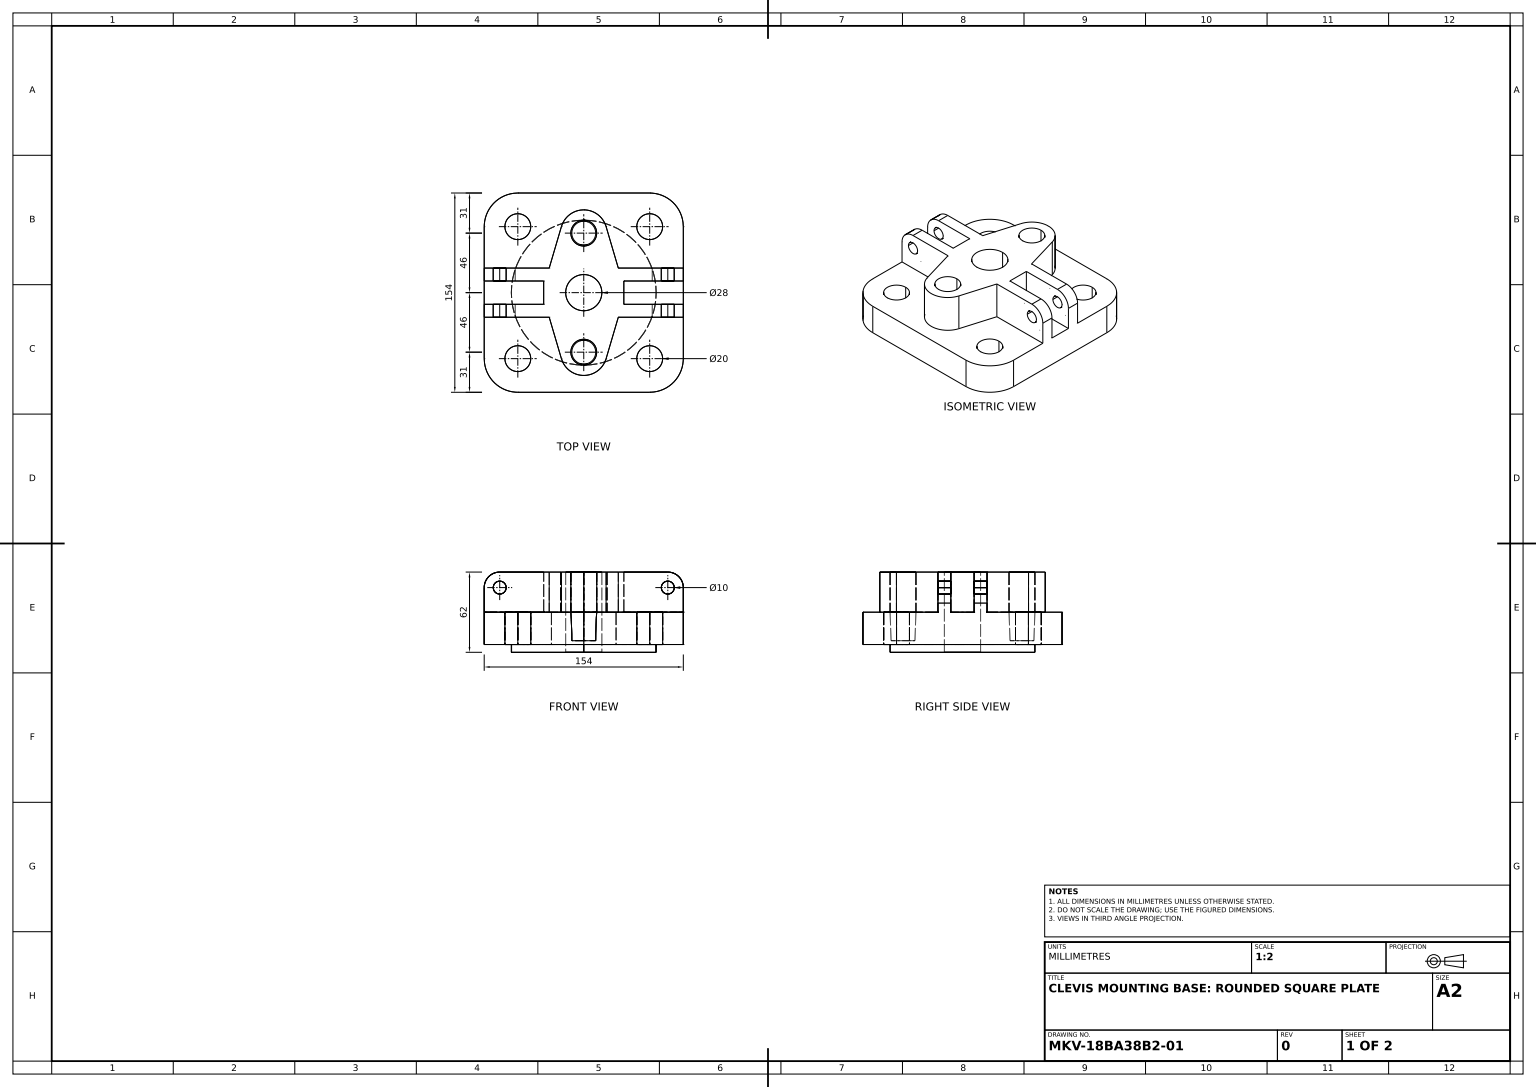
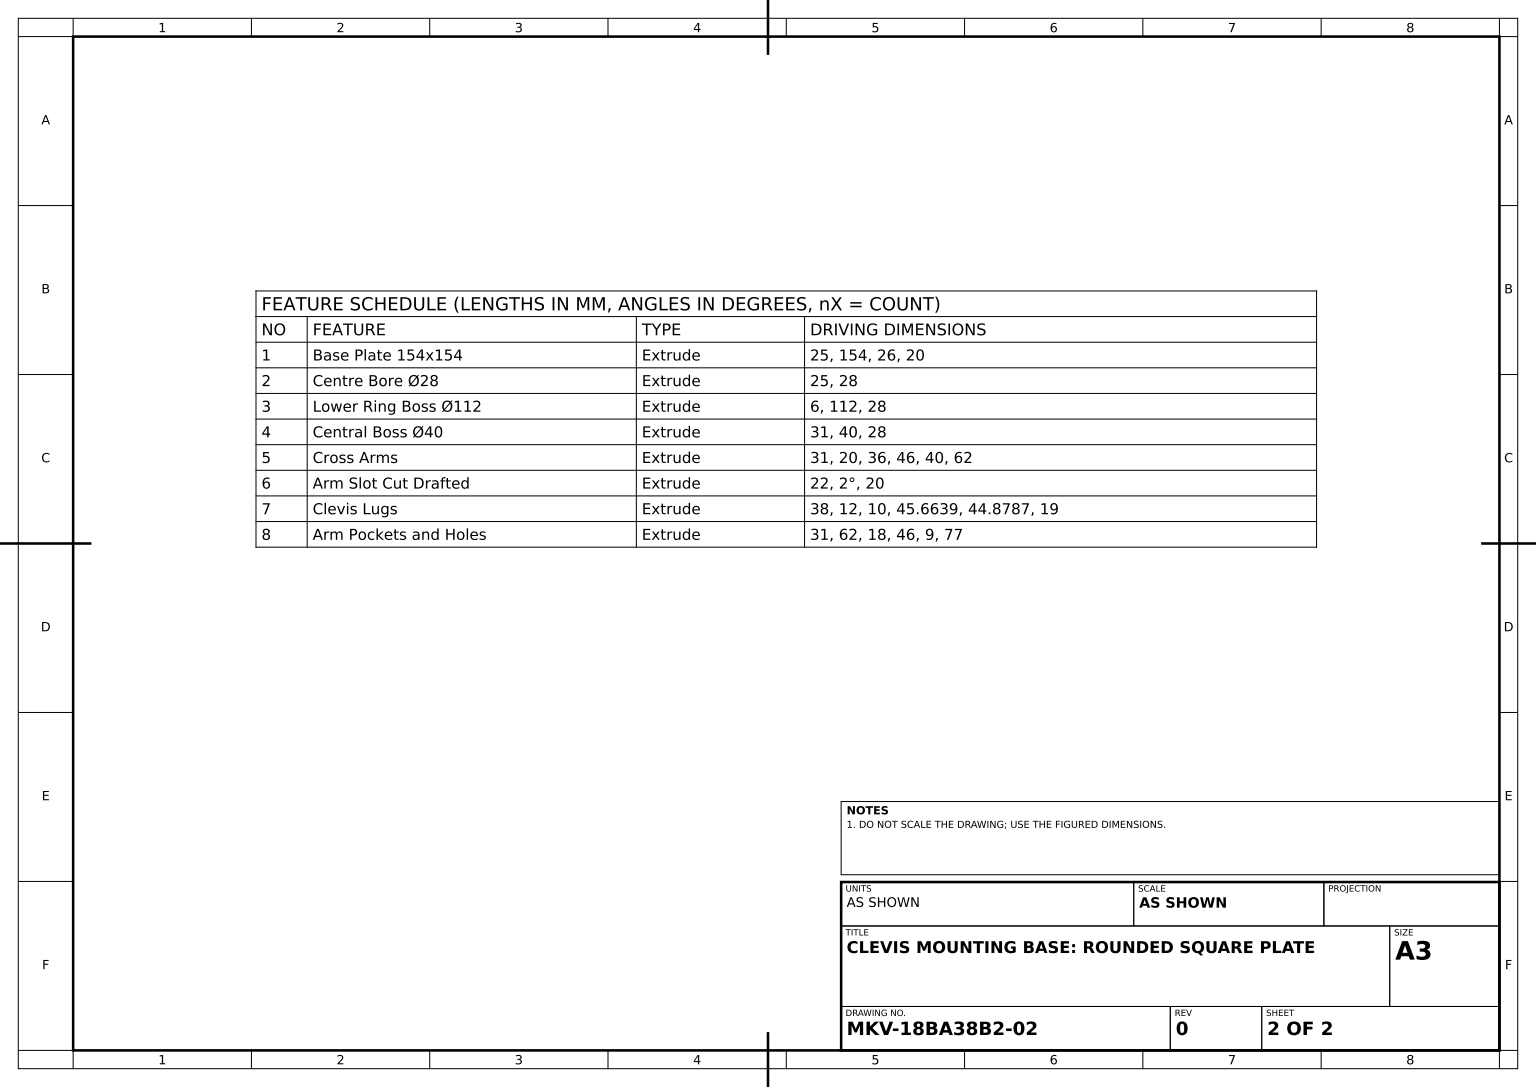
solid
v1 (0,56,-36)
v2 (0,56,-56)
e1 v1 v2 CIRCLE(AX(P(0,56,-46),D(0,1,0),D(0,0,1)),10)
v3 (0,25,-56)
e2 v2 v3 LINE
v4 (0,25,-36)
e3 v4 v3 CIRCLE(AX(P(0,25,-46),D(0,1,0),D(0,0,1)),10)
e4 v1 v4 LINE
face CYL(AX(P(0,56,-46),D(0,-1,0),D(0,0,-1)),10) rev [e1 e2 -e3 -e4]
v5 (-31,25,9)
v6 (-31,25,-9)
e5 v5 v6 LINE
v7 (-77,25,-9)
e6 v7 v6 LINE
v8 (-77,25,9)
e7 v7 v8 LINE
e8 v8 v5 LINE
face PLANE(AX(P(0,25,0),D(0,1,0),D(0,0,1))) [e5 -e6 e7 e8]
v9 (60,44,-9)
v10 (70,44,-9)
e9 v9 v10 CIRCLE(AX(P(65,44,-9),D(0,0,1),D(1,0,0)),5)
v11 (70,44,-19)
e10 v10 v11 LINE
v12 (60,44,-19)
e11 v12 v11 CIRCLE(AX(P(65,44,-19),D(0,0,1),D(1,0,0)),5)
e12 v9 v12 LINE
face CYL(AX(P(65,44,19),D(0,0,-1),D(-1,0,0)),5) rev [e9 e10 -e11 -e12]
v13 (-31,56,9)
e13 v5 v13 LINE
v14 (-31,56,-9)
e14 v13 v14 LINE
e15 v6 v14 LINE
face PLANE(AX(P(-31,25,0),D(1,0,0),D(0,0,-1))) rev [-e5 e13 e14 -e15]
v15 (17.266235,56,-51.086957)
v16 (0,56,-64)
e16 v15 v16 CIRCLE(AX(P(0,56,-46),D(0,1,0),D(0,0,1)),18)
v17 (17.266235,25,-51.086957)
e17 v15 v17 LINE
v18 (0,25,-64)
e18 v17 v18 CIRCLE(AX(P(0,25,-46),D(0,1,0),D(0,0,1)),18)
e19 v16 v18 LINE
face CYL(AX(P(0,56,-46),D(0,-1,0),D(0,0,-1)),18) [-e16 e17 e18 -e19]
v19 (31,25,-9)
v20 (77,25,-9)
e20 v19 v20 LINE
v21 (77,44,-9)
e21 v20 v21 LINE
v22 (65,56,-9)
e22 v21 v22 CIRCLE(AX(P(65,44,-9),D(0,0,1),D(1,0,0)),12)
v23 (31,56,-9)
e23 v23 v22 LINE
e24 v19 v23 LINE
e25 v10 v9 CIRCLE(AX(P(65,44,-9),D(0,0,1),D(1,0,0)),5)
face PLANE(AX(P(0,25,-9),D(0,0,1),D(1,0,0))) [e20 e21 e22 -e23 -e24] [-e9 -e25]
v24 (-60,44,9)
v25 (-70,44,9)
e26 v24 v25 CIRCLE(AX(P(-65,44,9),D(0,0,1),D(1,0,0)),5)
v26 (-60,44,19)
e27 v26 v24 LINE
v27 (-70,44,19)
e28 v26 v27 CIRCLE(AX(P(-65,44,19),D(0,0,1),D(1,0,0)),5)
e29 v27 v25 LINE
face CYL(AX(P(-65,44,19),D(0,0,-1),D(-1,0,0)),5) rev [-e26 -e27 e28 e29]
v28 (77,25,9)
e30 v20 v28 LINE
v29 (77,44,9)
e31 v28 v29 LINE
v30 (77,44,19)
e32 v30 v29 LINE
v31 (77,25,19)
e33 v31 v30 LINE
v32 (77,25,51)
e34 v32 v31 LINE
v33 (77,0,51)
e35 v32 v33 LINE
v34 (77,0,-51)
e36 v33 v34 LINE
v35 (77,25,-51)
e37 v35 v34 LINE
v36 (77,25,-19)
e38 v36 v35 LINE
v37 (77,44,-19)
e39 v36 v37 LINE
e40 v21 v37 LINE
face PLANE(AX(P(77,25,-51),D(-1,0,0),D(0,0,1))) rev [e30 e31 -e32 -e33 -e34 e35 e36 -e37 -e38 e39 -e40 -e21]
e41 v11 v12 CIRCLE(AX(P(65,44,-19),D(0,0,1),D(1,0,0)),5)
face CYL(AX(P(65,44,19),D(0,0,-1),D(-1,0,0)),5) rev [e25 e12 -e41 -e10]
v38 (-17.266235,56,-51.086957)
v39 (-17.266235,25,-51.086957)
e42 v38 v39 LINE
e43 v16 v38 CIRCLE(AX(P(0,56,-46),D(0,1,0),D(0,0,1)),18)
e44 v18 v39 CIRCLE(AX(P(0,25,-46),D(0,1,0),D(0,0,1)),18)
face CYL(AX(P(0,56,-46),D(0,-1,0),D(0,0,-1)),18) [-e42 -e43 e19 e44]
v40 (51,25,-61)
v41 (51,0,-61)
e45 v40 v41 LINE
v42 (51,25,-41)
e46 v40 v42 CIRCLE(AX(P(51,25,-51),D(0,1,0),D(0,0,1)),10)
v43 (51,0,-41)
e47 v42 v43 LINE
e48 v41 v43 CIRCLE(AX(P(51,0,-51),D(0,1,0),D(0,0,1)),10)
face CYL(AX(P(51,25,-51),D(0,-1,0),D(0,0,-1)),10) rev [-e45 e46 e47 -e48]
v44 (60,44,19)
v45 (60,44,9)
e49 v44 v45 LINE
v46 (70,44,19)
e50 v44 v46 CIRCLE(AX(P(65,44,19),D(0,0,1),D(1,0,0)),5)
v47 (70,44,9)
e51 v46 v47 LINE
e52 v45 v47 CIRCLE(AX(P(65,44,9),D(0,0,1),D(1,0,0)),5)
face CYL(AX(P(65,44,19),D(0,0,-1),D(-1,0,0)),5) rev [-e49 e50 e51 -e52]
v48 (0,-6,-56)
v49 (0,-6,56)
e53 v48 v49 CIRCLE(AX(P(0,-6,0),D(0,-1,0),D(0,0,-1)),56)
e54 v49 v48 CIRCLE(AX(P(0,-6,0),D(0,-1,0),D(0,0,-1)),56)
v50 (0,-6,-14)
v51 (0,-6,14)
e55 v50 v51 CIRCLE(AX(P(0,-6,0),D(0,-1,0),D(0,0,-1)),14)
e56 v51 v50 CIRCLE(AX(P(0,-6,0),D(0,-1,0),D(0,0,-1)),14)
face PLANE(AX(P(0,-6,0),D(0,-1,0),D(0,0,-1))) [e53 e54] [-e55 -e56]
v52 (17.266235,56,51.086957)
v53 (17.266235,25,51.086957)
e57 v52 v53 LINE
v54 (-17.266235,56,51.086957)
e58 v54 v52 CIRCLE(AX(P(0,56,46),D(0,1,0),D(0,0,1)),18)
v55 (-17.266235,25,51.086957)
e59 v54 v55 LINE
e60 v55 v53 CIRCLE(AX(P(0,25,46),D(0,1,0),D(0,0,1)),18)
face CYL(AX(P(0,56,46),D(0,-1,0),D(0,0,-1)),18) [-e57 -e58 e59 e60]
v56 (-60,44,-19)
v57 (-70,44,-19)
e61 v56 v57 CIRCLE(AX(P(-65,44,-19),D(0,0,1),D(1,0,0)),5)
e62 v57 v56 CIRCLE(AX(P(-65,44,-19),D(0,0,1),D(1,0,0)),5)
v58 (-77,25,-19)
v59 (-26.719654,25,-19)
e63 v58 v59 LINE
v60 (-77,44,-19)
e64 v60 v58 LINE
v61 (-65,56,-19)
e65 v61 v60 CIRCLE(AX(P(-65,44,-19),D(0,0,1),D(1,0,0)),12)
v62 (-26.719654,56,-19)
e66 v62 v61 LINE
e67 v62 v59 LINE
face PLANE(AX(P(-65,44,-19),D(0,0,1),D(1,0,0))) rev [e61 e62] [-e63 -e64 -e65 -e66 e67]
v63 (51,25,41)
v64 (51,0,41)
e68 v63 v64 LINE
v65 (51,25,61)
e69 v63 v65 CIRCLE(AX(P(51,25,51),D(0,1,0),D(0,0,1)),10)
v66 (51,0,61)
e70 v65 v66 LINE
e71 v64 v66 CIRCLE(AX(P(51,0,51),D(0,1,0),D(0,0,1)),10)
face CYL(AX(P(51,25,51),D(0,-1,0),D(0,0,-1)),10) rev [-e68 e69 e70 -e71]
e72 v65 v63 CIRCLE(AX(P(51,25,51),D(0,1,0),D(0,0,1)),10)
e73 v66 v64 CIRCLE(AX(P(51,0,51),D(0,1,0),D(0,0,1)),10)
face CYL(AX(P(51,25,51),D(0,-1,0),D(0,0,-1)),10) rev [e72 e68 -e73 -e70]
e74 v27 v26 CIRCLE(AX(P(-65,44,19),D(0,0,1),D(1,0,0)),5)
e75 v25 v24 CIRCLE(AX(P(-65,44,9),D(0,0,1),D(1,0,0)),5)
face CYL(AX(P(-65,44,19),D(0,0,-1),D(-1,0,0)),5) rev [-e29 e74 e27 -e75]
v67 (-51,25,-41)
v68 (-51,0,-41)
e76 v67 v68 LINE
v69 (-51,25,-61)
e77 v67 v69 CIRCLE(AX(P(-51,25,-51),D(0,1,0),D(0,0,1)),10)
v70 (-51,0,-61)
e78 v69 v70 LINE
e79 v68 v70 CIRCLE(AX(P(-51,0,-51),D(0,1,0),D(0,0,1)),10)
face CYL(AX(P(-51,25,-51),D(0,-1,0),D(0,0,-1)),10) rev [-e76 e77 e78 -e79]
v71 (31,25,9)
e80 v71 v19 LINE
e81 v71 v28 LINE
face PLANE(AX(P(0,25,0),D(0,1,0),D(0,0,1))) [-e30 -e20 -e80 e81]
v72 (-60,44,-9)
e82 v72 v56 LINE
v73 (-70,44,-9)
e83 v72 v73 CIRCLE(AX(P(-65,44,-9),D(0,0,1),D(1,0,0)),5)
e84 v73 v57 LINE
face CYL(AX(P(-65,44,19),D(0,0,-1),D(-1,0,0)),5) rev [-e61 -e82 e83 e84]
e85 v70 v68 CIRCLE(AX(P(-51,0,-51),D(0,1,0),D(0,0,1)),10)
e86 v69 v67 CIRCLE(AX(P(-51,25,-51),D(0,1,0),D(0,0,1)),10)
face CYL(AX(P(-51,25,-51),D(0,-1,0),D(0,0,-1)),10) rev [e76 -e85 -e78 e86]
v74 (31,56,9)
e87 v71 v74 LINE
e88 v74 v23 LINE
face PLANE(AX(P(31,25,0),D(1,0,0),D(0,0,-1))) [-e87 e80 e24 -e88]
v75 (0,56,36)
v76 (0,25,36)
e89 v75 v76 LINE
v77 (0,56,56)
e90 v75 v77 CIRCLE(AX(P(0,56,46),D(0,1,0),D(0,0,1)),10)
v78 (0,25,56)
e91 v77 v78 LINE
e92 v76 v78 CIRCLE(AX(P(0,25,46),D(0,1,0),D(0,0,1)),10)
face CYL(AX(P(0,56,46),D(0,-1,0),D(0,0,-1)),10) rev [-e89 e90 e91 -e92]
e93 v3 v4 CIRCLE(AX(P(0,25,-46),D(0,1,0),D(0,0,1)),10)
v79 (0,3,-36.768257)
e94 v79 v4 LINE
v80 (0,3,-55.231743)
e95 v80 v79 CIRCLE(AX(P(0,3,-46),D(0,1,0),D(0,0,1)),9.231743)
e96 v80 v3 LINE
face CONE(AX(P(0,25,-46),D(0,1,0),D(0,0,1)),10,0.034906585) rev [e93 -e94 -e95 e96]
v81 (0,3,55.231743)
e97 v81 v78 LINE
v82 (0,3,36.768257)
e98 v82 v81 CIRCLE(AX(P(0,3,46),D(0,1,0),D(0,0,1)),9.231743)
e99 v82 v76 LINE
face CONE(AX(P(0,25,46),D(0,1,0),D(0,0,1)),10,0.034906585) rev [e92 -e97 -e98 e99]
v83 (26.719654,25,-19)
v84 (26.719654,56,-19)
e100 v83 v84 LINE
v85 (65,56,-19)
e101 v85 v84 LINE
e102 v37 v85 CIRCLE(AX(P(65,44,-19),D(0,0,1),D(1,0,0)),12)
e103 v83 v36 LINE
face PLANE(AX(P(65,44,-19),D(0,0,1),D(1,0,0))) rev [e11 e41] [e100 -e101 -e102 -e39 -e103]
v86 (-51,25,61)
v87 (-51,0,61)
e104 v86 v87 LINE
v88 (-51,0,41)
e105 v88 v87 CIRCLE(AX(P(-51,0,51),D(0,1,0),D(0,0,1)),10)
v89 (-51,25,41)
e106 v89 v88 LINE
e107 v89 v86 CIRCLE(AX(P(-51,25,51),D(0,1,0),D(0,0,1)),10)
face CYL(AX(P(-51,25,51),D(0,-1,0),D(0,0,-1)),10) rev [e104 -e105 -e106 e107]
v90 (0,0,56)
e108 v49 v90 LINE
v91 (0,0,-56)
e109 v90 v91 CIRCLE(AX(P(0,0,0),D(0,-1,0),D(0,0,-1)),56)
e110 v48 v91 LINE
face CYL(AX(P(0,-6,0),D(0,1,0),D(0,0,1)),56) [-e54 e108 e109 -e110]
v92 (65,56,9)
e111 v74 v92 LINE
e112 v29 v92 CIRCLE(AX(P(65,44,9),D(0,0,1),D(1,0,0)),12)
e113 v47 v45 CIRCLE(AX(P(65,44,9),D(0,0,1),D(1,0,0)),5)
face PLANE(AX(P(0,25,9),D(0,0,1),D(1,0,0))) rev [e111 -e112 -e31 -e81 e87] [e113 e52]
e114 v22 v85 LINE
face CYL(AX(P(65,44,19),D(0,0,-1),D(-1,0,0)),12) [e40 e102 -e114 -e22]
e115 v91 v90 CIRCLE(AX(P(0,0,0),D(0,-1,0),D(0,0,-1)),56)
face CYL(AX(P(0,-6,0),D(0,1,0),D(0,0,1)),56) [-e108 -e53 e110 e115]
v93 (-51,0,-77)
v94 (-77,0,-51)
e116 v93 v94 CIRCLE(AX(P(-51,0,-51),D(0,1,0),D(0,0,1)),26)
v95 (-77,25,-51)
e117 v95 v94 LINE
v96 (-51,25,-77)
e118 v96 v95 CIRCLE(AX(P(-51,25,-51),D(0,1,0),D(0,0,1)),26)
e119 v96 v93 LINE
face CYL(AX(P(-51,25,-51),D(0,-1,0),D(0,0,-1)),26) [e116 -e117 -e118 e119]
e120 v73 v72 CIRCLE(AX(P(-65,44,-9),D(0,0,1),D(1,0,0)),5)
face CYL(AX(P(-65,44,19),D(0,0,-1),D(-1,0,0)),5) rev [e120 e82 -e62 -e84]
v97 (51,25,-77)
e121 v35 v97 CIRCLE(AX(P(51,25,-51),D(0,1,0),D(0,0,-1)),26)
v98 (51,0,-77)
e122 v34 v98 CIRCLE(AX(P(51,0,-51),D(0,1,0),D(0,0,-1)),26)
e123 v97 v98 LINE
face CYL(AX(P(51,25,-51),D(0,-1,0),D(0,0,-1)),26) [-e121 e37 e122 -e123]
v99 (-65,56,19)
v100 (-65,56,9)
e124 v99 v100 LINE
v101 (-77,44,9)
e125 v100 v101 CIRCLE(AX(P(-65,44,9),D(0,0,1),D(1,0,0)),12)
v102 (-77,44,19)
e126 v102 v101 LINE
e127 v99 v102 CIRCLE(AX(P(-65,44,19),D(0,0,1),D(1,0,0)),12)
face CYL(AX(P(-65,44,19),D(0,0,-1),D(-1,0,0)),12) [e124 e125 -e126 -e127]
v103 (-77,44,-9)
e128 v103 v60 LINE
v104 (-65,56,-9)
e129 v104 v103 CIRCLE(AX(P(-65,44,-9),D(0,0,1),D(1,0,0)),12)
e130 v104 v61 LINE
face CYL(AX(P(-65,44,19),D(0,0,-1),D(-1,0,0)),12) [-e128 -e129 e130 e65]
v105 (65,56,19)
e131 v105 v92 LINE
e132 v30 v105 CIRCLE(AX(P(65,44,19),D(0,0,1),D(1,0,0)),12)
face CYL(AX(P(65,44,19),D(0,0,-1),D(-1,0,0)),12) [e32 e112 -e131 -e132]
v106 (26.719654,25,19)
v107 (26.719654,56,19)
e133 v106 v107 LINE
e134 v52 v107 LINE
e135 v53 v106 LINE
face PLANE(AX(P(17.266235,56,51.086957),D(-0.959235281,0,-0.282608696),D(-0.282608696,0,0.959235281))) rev [e133 -e134 e57 e135]
v108 (-26.719654,56,19)
v109 (-26.719654,25,19)
e136 v108 v109 LINE
e137 v108 v99 LINE
v110 (-77,25,19)
e138 v102 v110 LINE
e139 v110 v109 LINE
face PLANE(AX(P(-65,44,19),D(0,0,1),D(1,0,0))) [-e136 e137 e127 e138 e139] [-e74 -e28]
e140 v95 v58 LINE
v111 (-77,0,51)
e141 v94 v111 LINE
v112 (-77,25,51)
e142 v112 v111 LINE
e143 v110 v112 LINE
e144 v8 v101 LINE
e145 v7 v103 LINE
face PLANE(AX(P(-77,25,-51),D(1,0,0),D(0,0,-1))) rev [e64 -e140 e117 e141 -e142 -e143 -e138 e126 -e144 -e7 e145 e128]
e146 v83 v17 LINE
e147 v84 v15 LINE
face PLANE(AX(P(29.736294,56,-8.76087),D(-0.959235281,0,0.282608696),D(0.282608696,0,0.959235281))) rev [-e100 e146 -e17 -e147]
e148 v79 v80 CIRCLE(AX(P(0,3,-46),D(0,1,0),D(0,0,1)),9.231743)
face PLANE(AX(P(0,3,-46),D(0,1,0),D(0,0,1))) [e148 e95]
v113 (0,56,14)
v114 (0,56,-14)
e149 v113 v114 CIRCLE(AX(P(0,56,0),D(0,1,0),D(0,0,1)),14)
e150 v114 v113 CIRCLE(AX(P(0,56,0),D(0,1,0),D(0,0,1)),14)
e151 v2 v1 CIRCLE(AX(P(0,56,-46),D(0,1,0),D(0,0,1)),10)
e152 v104 v14 LINE
e153 v100 v13 LINE
e154 v108 v54 LINE
e155 v105 v107 LINE
e156 v38 v62 LINE
e157 v77 v75 CIRCLE(AX(P(0,56,46),D(0,1,0),D(0,0,1)),10)
face PLANE(AX(P(0,56,0),D(0,1,0),D(0,0,1))) [-e149 -e150] [-e151 -e1] [e66 -e130 e152 -e14 -e153 -e124 -e137 e154 e58 e134 -e155 e131 -e111 e88 e23 e114 e101 e147 e16 e43 e156] [-e90 -e157]
v115 (-51,25,77)
v116 (-51,0,77)
e158 v115 v116 LINE
v117 (51,0,77)
e159 v116 v117 LINE
v118 (51,25,77)
e160 v118 v117 LINE
e161 v115 v118 LINE
face PLANE(AX(P(-51,25,77),D(0,0,-1),D(-1,0,0))) rev [e158 e159 -e160 -e161]
e162 v98 v93 LINE
e163 v97 v96 LINE
face PLANE(AX(P(-51,25,-77),D(0,0,1),D(1,0,0))) rev [e123 e162 -e119 -e163]
e164 v87 v88 CIRCLE(AX(P(-51,0,51),D(0,1,0),D(0,0,1)),10)
e165 v86 v89 CIRCLE(AX(P(-51,25,51),D(0,1,0),D(0,0,1)),10)
face CYL(AX(P(-51,25,51),D(0,-1,0),D(0,0,-1)),10) rev [-e164 -e104 e165 e106]
e166 v117 v33 CIRCLE(AX(P(51,0,51),D(0,1,0),D(0,0,1)),26)
e167 v118 v32 CIRCLE(AX(P(51,25,51),D(0,1,0),D(0,0,1)),26)
face CYL(AX(P(51,25,51),D(0,-1,0),D(0,0,-1)),26) [e166 -e35 -e167 e160]
e168 v111 v116 CIRCLE(AX(P(-51,0,51),D(0,1,0),D(0,0,1)),26)
e169 v43 v41 CIRCLE(AX(P(51,0,-51),D(0,1,0),D(0,0,1)),10)
face PLANE(AX(P(51,0,51),D(0,1,0),D(0,0,1))) rev [e71 e73] [-e141 -e116 -e162 -e122 -e36 -e166 -e159 -e168] [e79 e85] [e105 e164] [e48 e169] [-e115 -e109]
e170 v81 v82 CIRCLE(AX(P(0,3,46),D(0,1,0),D(0,0,1)),9.231743)
face PLANE(AX(P(0,3,46),D(0,1,0),D(0,0,1))) [e98 e170]
e171 v50 v114 LINE
e172 v51 v113 LINE
face CYL(AX(P(0,0,0),D(0,1,0),D(0,0,1)),14) rev [-e171 e55 e172 e149]
e173 v42 v40 CIRCLE(AX(P(51,25,-51),D(0,1,0),D(0,0,1)),10)
e174 v39 v59 LINE
face PLANE(AX(P(51,25,51),D(0,1,0),D(0,0,1))) [-e46 -e173] [-e77 -e86] [e121 e163 e118 e140 e63 -e174 -e44 -e18 -e146 e103 e38]
e175 v112 v115 CIRCLE(AX(P(-51,25,51),D(0,1,0),D(0,0,1)),26)
face CYL(AX(P(-51,25,51),D(0,-1,0),D(0,0,-1)),26) [e142 e168 -e158 -e175]
face PLANE(AX(P(0,25,9),D(0,0,1),D(1,0,0))) rev [e26 e75] [-e125 e153 -e13 -e8 e144]
face PLANE(AX(P(0,25,-9),D(0,0,1),D(1,0,0))) [e129 -e145 e6 e15 -e152] [-e120 -e83]
face PLANE(AX(P(-29.736294,56,-8.76087),D(0.959235281,0,0.282608696),D(0.282608696,0,-0.959235281))) rev [e174 -e67 -e156 e42]
face CYL(AX(P(0,0,0),D(0,1,0),D(0,0,1)),14) rev [-e172 e56 e171 e150]
face CYL(AX(P(0,56,-46),D(0,-1,0),D(0,0,-1)),10) rev [e151 e4 -e93 -e2]
e176 v46 v44 CIRCLE(AX(P(65,44,19),D(0,0,1),D(1,0,0)),5)
face CYL(AX(P(65,44,19),D(0,0,-1),D(-1,0,0)),5) rev [e176 e49 -e113 -e51]
face CYL(AX(P(51,25,-51),D(0,-1,0),D(0,0,-1)),10) rev [-e47 e173 e45 -e169]
e177 v78 v76 CIRCLE(AX(P(0,25,46),D(0,1,0),D(0,0,1)),10)
face CYL(AX(P(0,56,46),D(0,-1,0),D(0,0,-1)),10) rev [-e91 e157 e89 -e177]
e178 v109 v55 LINE
face PLANE(AX(P(-29.736294,56,8.76087),D(0.959235281,0,-0.282608696),D(-0.282608696,0,-0.959235281))) rev [e178 -e59 -e154 e136]
e179 v106 v31 LINE
face PLANE(AX(P(65,44,19),D(0,0,1),D(1,0,0))) [e155 -e133 e179 e33 e132] [-e176 -e50]
face CONE(AX(P(0,25,-46),D(0,1,0),D(0,0,1)),10,0.034906585) rev [e3 -e96 -e148 e94]
face PLANE(AX(P(51,25,51),D(0,1,0),D(0,0,1))) [e167 e34 -e179 -e135 -e60 -e178 -e139 e143 e175 e161] [-e107 -e165] [-e69 -e72]
face CONE(AX(P(0,25,46),D(0,1,0),D(0,0,1)),10,0.034906585) rev [-e99 -e170 e97 e177]
